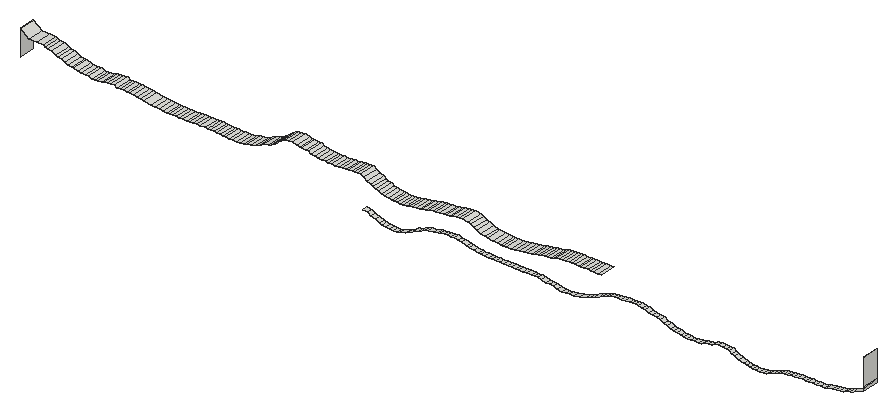
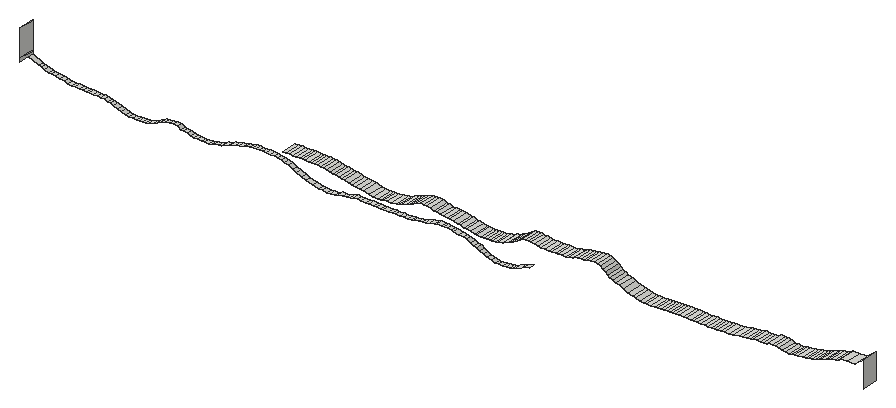
# SketchUp Ruby script. Lengths in inches.
U = 1.inch
M = Sketchup.active_model
def pt(a) = Geom::Point3d.new(a.map { |v| v * U })
def face(e, loops, mat)
  f = e.add_face(loops[0].map { |a| pt(a) })
  loops[1..].each { |l| e.add_face(l.map { |a| pt(a) }).erase! }
  f.material = f.back_material = mat if mat
  f
end
# faces: each face lists its corners as indices into pts; further lists are holes
def faces(e, pts, list, mat = nil) = list.each { |f| face(e, (f[0].is_a?(Array) ? f : [f]).map { |l| l.map { |i| pts[i] } }, mat) }
# xy, xz, yz: faces in a plane at the given z, y or x. An outline is a flat list of corners, or four numbers for a rectangle; further outlines are holes
def ring(l) = l.size == 4 ? [[l[0], l[1]], [l[2], l[1]], [l[2], l[3]], [l[0], l[3]]] : l.each_slice(2).to_a
def flat(e, list, mat, &to3) = list.each { |f| face(e, (f[0].is_a?(Array) ? f : [f]).map { |l| ring(l).map { |u, v| to3.(u, v) } }, mat) }
def xy(e, z, list, mat = nil) = flat(e, list, mat) { |x, y| [x, y, z] }
def xz(e, y, list, mat = nil) = flat(e, list, mat) { |x, z| [x, y, z] }
def yz(e, x, list, mat = nil) = flat(e, list, mat) { |y, z| [x, y, z] }
def lines(e, pts, list) = list.each { |a, b| e.add_line(pt(pts[a]), pt(pts[b])) }
# prism: a flat outline (further loops are holes) pulled along v
def prism(e, loops, v, mat = nil)
  f = face(e, loops, mat); d = Geom::Vector3d.new(v.map { |x| x * U })
  f.pushpull(f.normal.samedirection?(d) ? d.length : -d.length)
end
def box(e, o, s, mat = nil) = prism(e, [[o, [o[0] + s[0], o[1], o[2]], [o[0] + s[0], o[1] + s[1], o[2]], [o[0], o[1] + s[1], o[2]]]], [0, 0, s[2]], mat)
def at(x, y, z, deg = 0) = Geom::Transformation.translation(pt([x, y, z])) * Geom::Transformation.rotation(ORIGIN, Z_AXIS, deg.degrees)
def axes(o, x, y, z) = Geom::Transformation.new([*x, 0, *y, 0, *z, 0, *pt(o).to_a, 1])
def part(name) = M.definitions.add(name)
# library, detail: a bought-in or finely detailed component or shape, given as its bounding box
def library(name, o, s) = part(name).tap { |d| box(d.entities, o, s) }
def detail(e, o, s) = box(e.add_group.entities, o, s)
def put(e, d, t, mat = nil) = e.add_instance(d, t).tap { |i| i.material = mat if mat }
def group(e, t, mat = nil) = e.add_group.tap { |g| g.transformation = t; g.material = mat if mat }.entities
root = M.entities
xy(root,238.18,[[1254.78,565.74,1255.46,566.68]])
xy(root,238.62,[[1221.31,565.74,1222.08,566.68],[1222.08,565.74,1222.71,566.68],[1222.71,565.74,1223.47,566.68],[1223.47,565.74,1224.09,566.68],[1224.09,565.74,1224.94,566.68],
  [1224.94,565.74,1225.58,566.68],[1225.58,565.74,1226.2,566.68]])
xy(root,238.625,[[1219.89,565.74,1220.75,566.68]])
xy(root,238.89,[[1275.7,565.74,1276.38,566.68]])
xy(root,238.9,[[1277.14,565.74,1277.76,566.68],[1277.76,565.74,1278.53,566.68]])
xy(root,240.43,[[1243.98,565.74,1244.55,566.68]])
xy(root,241.68,[[1162.03,565.74,1162.62,568.68]])
xy(root,241.75,[[1164.38,565.74,1165.25,568.68],[1165.25,565.74,1165.87,568.68],[1165.87,565.74,1166.38,568.68]])
xy(root,243.05,[[1237.04,565.74,1237.72,568.68]])
xy(root,243.07,[[1235.1875,565.74,1235.77,568.68]])
xy(root,243.09,[[1231.875,565.74,1232.4,568.68],[1232.4,565.74,1232.92,568.68],[1232.92,565.74,1233.58,568.68],[1233.58,565.74,1234.03,568.68]])
yz(root,1131.59,[[565.74,241.52,568.68,246.2]])
yz(root,1285.6,[[565.74,240.89,565.74,241.29,568.68,241.52,568.68,240.89],[565.74,241.29,568.68,241.52,565.74,241.52],[565.74,241.52,565.74,246.27,566.4375,246.36,568.68,246.43,568.68,241.52],[565.74,246.27,565.74,246.43,568.68,246.43,566.4375,246.36]])
p = [[1198.39,565.74,237.11],[1198.39,566.68,237.11],[1199.15,566.68,237.04],[1199.15,565.74,237.04],[1199.84,566.68,237.01],[1199.84,565.74,237.01],
  [1200.45,566.68,236.98],[1200.45,565.74,236.98],[1201.13,566.68,237.22],[1201.13,565.74,237.22],[1197.7,565.74,237.2],[1197.7,566.68,237.2],
  [1197.17,565.74,237.33],[1197.17,566.68,237.33],[1201.98,566.68,237.43],[1201.98,565.74,237.43],[1196.5,565.74,237.68],[1196.5,566.68,237.68],
  [1202.6,566.68,237.74],[1202.6,565.74,237.74],[1265.43,565.74,237.45],[1265.43,566.68,237.45],[1266,566.68,237.42],[1266,565.74,237.42],
  [1266.73,566.68,237.4],[1266.73,565.74,237.4],[1267.41,566.68,237.47],[1267.41,565.74,237.47],[1264.24,565.74,237.59],[1264.24,566.68,237.59],
  [1264.84,566.68,237.51],[1264.84,565.74,237.51],[1268.01,566.68,237.5625],[1268.01,565.74,237.5625],[1263.7,565.74,237.71],[1263.7,566.68,237.71],
  [1268.7,566.68,237.84],[1268.7,565.74,237.84],[1195.5625,565.74,237.96],[1195.5625,566.68,237.96],[1203.3,566.68,238.02],[1203.3,565.74,238.02],
  [1230.44,565.74,237.79],[1230.44,566.68,237.79],[1231.15,566.68,237.74],[1231.15,565.74,237.74],[1232.02,566.68,237.87],[1232.02,565.74,237.87],
  [1262.87,565.74,238],[1262.87,566.68,238],[1229.67,565.74,237.86],[1229.67,566.68,237.86],[1269.38,566.68,238.08],[1269.38,565.74,238.08],
  [1229.04,565.74,238.15],[1229.04,566.68,238.15],[1232.67,566.68,237.88],[1232.67,565.74,237.88],[1233.79,566.68,238.14],[1233.79,565.74,238.14],
  [1195,565.74,238.28],[1195,566.68,238.28],[1203.74,566.68,238.375],[1203.74,565.74,238.375],[1262.16,565.74,238.33],[1262.16,566.68,238.33],
  [1228.27,565.74,238.19],[1228.27,566.68,238.19],[1235.01,566.68,238.46],[1235.01,565.74,238.46],[1252.76,565.74,238.19],[1252.76,566.68,238.19],
  [1253.58,566.68,238.15],[1253.58,565.74,238.15],[1254.11,566.68,238.11],[1254.11,565.74,238.11],[1254.78,566.68,238.18],[1254.78,565.74,238.18],
  [1270.07,566.68,238.33],[1270.07,565.74,238.33],[1227.65,565.74,238.25],[1227.65,566.68,238.25],[1252.1875,565.74,238.26],[1252.1875,566.68,238.26],
  [1255.46,565.74,238.18],[1255.46,566.68,238.18],[1256.14,566.68,238.27],[1256.14,565.74,238.27],[1194.22,565.74,238.43],[1194.22,566.68,238.43],
  [1226.89,565.74,238.45],[1226.89,566.68,238.45],[1251.62,565.74,238.48],[1251.62,566.68,238.48],[1256.66,566.68,238.55],[1256.66,565.74,238.55],
  [1261.61,565.74,238.57],[1261.61,566.68,238.57],[1270.6,566.68,238.51],[1270.6,565.74,238.51],[1204.3,566.68,238.51],[1204.3,565.74,238.51],
  [1204.9375,566.68,238.76],[1204.9375,565.74,238.76],[1226.2,565.74,238.62],[1226.2,566.68,238.62],[1235.76,566.68,238.72],[1235.76,565.74,238.72],
  [1250.96,565.74,238.56],[1250.96,566.68,238.56],[1257.32,566.68,238.61],[1257.32,565.74,238.61],[1271.17,566.68,238.6],[1271.17,565.74,238.6],
  [1217.13,565.74,238.66],[1217.13,566.68,238.66],[1217.8,566.68,238.65],[1217.8,565.74,238.65],[1218.58,566.68,238.64],[1218.58,565.74,238.64],
  [1219.2,566.68,238.63],[1219.2,565.74,238.63],[1219.89,566.68,238.625],[1219.89,565.74,238.625],[1220.75,565.74,238.625],[1220.75,566.68,238.625],
  [1221.31,566.68,238.62],[1221.31,565.74,238.62],[1250.39,565.74,238.67],[1250.39,566.68,238.67],[1257.91,566.68,238.66],[1257.91,565.74,238.66],
  [1261.11,565.74,238.86],[1261.11,566.68,238.86],[1271.83,566.68,238.74],[1271.83,565.74,238.74],[1215.29,565.74,238.78],[1215.29,566.68,238.78],
  [1215.77,566.68,238.73],[1215.77,565.74,238.73],[1216.44,566.68,238.6875],[1216.44,565.74,238.6875],[1236.64,566.68,239.08],[1236.64,565.74,239.08],
  [1249.87,565.74,239.01],[1249.87,566.68,239.01],[1258.48,566.68,239.04],[1258.48,565.74,239.04],[1272.41,566.68,238.8],[1272.41,565.74,238.8],
  [1205.58,566.68,239.12],[1205.58,565.74,239.12],[1214.41,565.74,238.93],[1214.41,566.68,238.93],[1272.98,566.68,238.83],[1272.98,565.74,238.83],
  [1273.72,566.68,238.86],[1273.72,565.74,238.86],[1213.64,565.74,239.07],[1213.64,566.68,239.07],[1260.59,565.74,238.96],[1260.59,566.68,238.96],
  [1274.48,566.68,238.875],[1274.48,565.74,238.875],[1275.02,566.68,238.88],[1275.02,565.74,238.88],[1275.7,566.68,238.89],[1275.7,565.74,238.89],
  [1276.38,565.74,238.89],[1276.38,566.68,238.89],[1277.14,566.68,238.9],[1277.14,565.74,238.9],[1278.53,565.74,238.9],[1278.53,566.68,238.9],
  [1279.16,566.68,239.15],[1279.16,565.74,239.15],[1249.1875,565.74,239.18],[1249.1875,566.68,239.18],[1259.22,566.68,239.125],[1259.22,565.74,239.125],
  [1259.9,566.68,239.02],[1259.9,565.74,239.02],[1206.16,566.68,239.22],[1206.16,565.74,239.22],[1213.09,565.74,239.16],[1213.09,566.68,239.16],
  [1237.43,566.68,239.375],[1237.43,565.74,239.375],[1207.16,566.68,239.31],[1207.16,565.74,239.31],[1212.24,565.74,239.44],[1212.24,566.68,239.44],
  [1248.5625,565.74,239.5],[1248.5625,566.68,239.5],[1279.93,566.68,239.28],[1279.93,565.74,239.28],[1207.97,566.68,239.54],[1207.97,565.74,239.54],
  [1280.73,566.68,239.42],[1280.73,565.74,239.42],[1211.57,565.74,239.56],[1211.57,566.68,239.56],[1238.17,566.68,239.75],[1238.17,565.74,239.75],
  [1281.45,566.68,239.49],[1281.45,565.74,239.49],[1208.46,566.68,239.6],[1208.46,565.74,239.6],[1247.8,565.74,239.65],[1247.8,566.68,239.65],
  [1282,566.68,239.53],[1282,565.74,239.53],[1282.6875,566.68,239.81],[1282.6875,565.74,239.81],[1209.08,566.68,239.65],[1209.08,565.74,239.65],
  [1209.67,566.68,239.69],[1209.67,565.74,239.69],[1210.96,565.74,239.72],[1210.96,566.68,239.72],[1210.23,566.68,239.7],[1210.23,565.74,239.7],
  [1238.82,566.68,239.97],[1238.82,565.74,239.97],[1247.1875,565.74,239.8],[1247.1875,566.68,239.8],[1246.43,565.74,239.96],[1246.43,566.68,239.96],
  [1283.21,566.68,239.96],[1283.21,565.74,239.96],[1239.44,566.68,240.17],[1239.44,565.74,240.17],[1245.78,565.74,240.23],[1245.78,566.68,240.23],
  [1283.77,566.68,240.1],[1283.77,565.74,240.1],[1285.6,566.68,240.89],[1285.6,565.74,240.89],[1240.12,566.68,240.27],[1240.12,565.74,240.27],
  [1245.2,565.74,240.27],[1245.2,566.68,240.27],[1240.8,566.68,240.33],[1240.8,565.74,240.33],[1241.49,566.68,240.37],[1241.49,565.74,240.37],
  [1244.55,565.74,240.43],[1244.55,566.68,240.43],[1242.18,566.68,240.4],[1242.18,565.74,240.4],[1242.875,566.68,240.41],[1242.875,565.74,240.41],
  [1243.4,566.68,240.42],[1243.4,565.74,240.42],[1243.98,566.68,240.43],[1243.98,565.74,240.43],[1168.01,568.68,241.57],[1168.55,568.68,241.53],
  [1168.55,565.74,241.53],[1168.01,565.74,241.57],[1169.17,568.68,241.51],[1169.17,565.74,241.51],[1169.72,568.68,241.49],[1169.72,565.74,241.49],
  [1170.42,568.68,241.48],[1170.42,565.74,241.48],[1171.08,568.68,241.47],[1171.08,565.74,241.47],[1171.65,568.68,241.46],[1171.65,565.74,241.46],
  [1172.36,568.68,241.6],[1172.36,565.74,241.6],[1218.73,568.68,241.56],[1219.33,568.68,241.51],[1219.33,565.74,241.51],[1218.73,565.74,241.56],
  [1219.78,568.68,241.48],[1219.78,565.74,241.48],[1220.3,568.68,241.46],[1220.3,565.74,241.46],[1221.17,568.68,241.51],[1221.17,565.74,241.51],
  [1221.89,568.68,241.59],[1221.89,565.74,241.59],[1167.4,568.68,241.66],[1167.4,565.74,241.66],[1173.09,568.68,241.85],[1173.09,565.74,241.85],
  [1216.91,568.68,241.78],[1217.96,568.68,241.63],[1217.96,565.74,241.63],[1216.91,565.74,241.78],[1222.83,568.68,241.82],[1222.83,565.74,241.82],
  [1158.37,568.68,241.75],[1158.82,568.68,241.74],[1158.82,565.74,241.74],[1158.37,565.74,241.75],[1159.37,568.68,241.72],[1159.37,565.74,241.72],
  [1160,568.68,241.71],[1160,565.74,241.71],[1160.63,568.68,241.7],[1160.63,565.74,241.7],[1161.36,568.68,241.69],[1161.36,565.74,241.69],
  [1162.03,568.68,241.68],[1162.03,565.74,241.68],[1162.62,568.68,241.68],[1163.11,568.68,241.67],[1163.11,565.74,241.67],[1162.62,565.74,241.68],
  [1163.8125,568.68,241.74],[1163.8125,565.74,241.74],[1164.38,568.68,241.75],[1164.38,565.74,241.75],[1166.38,568.68,241.75],[1166.87,568.68,241.67],
  [1166.87,565.74,241.67],[1166.38,565.74,241.75],[1156.18,568.68,241.89],[1157,568.68,241.83],[1157,565.74,241.83],[1156.18,565.74,241.89],
  [1157.6,568.68,241.78],[1157.6,565.74,241.78],[1173.76,568.68,241.91],[1173.76,565.74,241.91],[1199.39,568.68,241.89],[1199.85,568.68,241.85],
  [1199.85,565.74,241.85],[1199.39,565.74,241.89],[1200.37,568.68,241.8125],[1200.37,565.74,241.8125],[1200.88,568.68,241.79],[1200.88,565.74,241.79],
  [1201.46,568.68,241.78],[1201.46,565.74,241.78],[1202.13,568.68,241.91],[1202.13,565.74,241.91],[1216.42,568.68,241.89],[1216.42,565.74,241.89],
  [1223.61,568.68,241.87],[1223.61,565.74,241.87],[1155.41,568.68,241.96],[1155.41,565.74,241.96],[1174.66,568.68,242.1],[1174.66,565.74,242.1],
  [1198.83,568.68,241.96],[1198.83,565.74,241.96],[1202.6,568.68,241.93],[1202.6,565.74,241.93],[1203.27,568.68,242.09],[1203.27,565.74,242.09],
  [1215.78,568.68,242.14],[1215.78,565.74,242.14],[1224.375,568.68,241.98],[1224.375,565.74,241.98],[1154.24,568.68,242.24],[1154.24,565.74,242.24],
  [1198.15,568.68,242.11],[1198.15,565.74,242.11],[1224.99,568.68,242.02],[1224.99,565.74,242.02],[1225.64,568.68,242.19],[1225.64,565.74,242.19],
  [1175.43,568.68,242.46],[1175.43,565.74,242.46],[1197.55,568.68,242.21],[1197.55,565.74,242.21],[1204.04,568.68,242.2],[1204.04,565.74,242.2],
  [1215.02,568.68,242.39],[1215.02,565.74,242.39],[1153.57,568.68,242.34],[1153.57,565.74,242.34],[1197.04,568.68,242.51],[1197.04,565.74,242.51],
  [1204.54,568.68,242.24],[1204.54,565.74,242.24],[1205.15,568.68,242.42],[1205.15,565.74,242.42],[1226.34,568.68,242.38],[1226.34,565.74,242.38],
  [1152.91,568.68,242.38],[1152.91,565.74,242.38],[1152.25,568.68,242.48],[1152.25,565.74,242.48],[1205.7,568.68,242.47],[1205.7,565.74,242.47],
  [1214.4,568.68,242.65],[1214.4,565.74,242.65],[1226.83,568.68,242.4375],[1226.83,565.74,242.4375],[1227.35,568.68,242.48],[1227.35,565.74,242.48],
  [1144.07,568.68,242.68],[1144.74,568.68,242.51],[1144.74,565.74,242.51],[1144.07,565.74,242.68],[1145.26,568.68,242.46],[1145.26,565.74,242.46],
  [1145.8,568.68,242.58],[1145.8,565.74,242.58],[1151.61,568.68,242.57],[1151.61,565.74,242.57],[1176.13,568.68,242.78],[1176.13,565.74,242.78],
  [1196.45,568.68,242.68],[1196.45,565.74,242.68],[1206.45,568.68,242.71],[1206.45,565.74,242.71],[1228.01,568.68,242.58],[1228.01,565.74,242.58],
  [1146.43,568.68,242.57],[1146.43,565.74,242.57],[1147.06,568.68,242.81],[1147.06,565.74,242.81],[1148.83,568.68,242.92],[1149.26,568.68,242.625],
  [1149.26,565.74,242.625],[1148.83,565.74,242.92],[1149.87,568.68,242.65],[1149.87,565.74,242.65],[1150.42,568.68,242.62],[1150.42,565.74,242.62],
  [1151.05,568.68,242.58],[1151.05,565.74,242.58],[1213.85,568.68,242.9375],[1213.85,565.74,242.9375],[1228.54,568.68,242.61],[1228.54,565.74,242.61],
  [1229.125,568.68,242.77],[1229.125,565.74,242.77],[1142.72,568.68,242.78],[1143.53,568.68,242.73],[1143.53,565.74,242.73],[1142.72,565.74,242.78],
  [1195.95,568.68,242.875],[1195.95,565.74,242.875],[1207.09,568.68,242.78],[1207.09,565.74,242.78],[1141.42,568.68,243.06],[1142.14,568.68,242.85],
  [1142.14,565.74,242.85],[1141.42,565.74,243.06],[1147.63,568.68,242.86],[1147.63,565.74,242.86],[1176.9,568.68,242.97],[1176.9,565.74,242.97],
  [1207.57,568.68,242.82],[1207.57,565.74,242.82],[1208.26,568.68,242.85],[1208.26,565.74,242.85],[1229.58,568.68,242.95],[1229.58,565.74,242.95],
  [1148.19,568.68,242.89],[1148.19,565.74,242.89],[1195.56,568.68,243.09],[1195.56,565.74,243.09],[1208.96,568.68,242.87],[1208.96,565.74,242.87],
  [1209.51,568.68,243.02],[1209.51,565.74,243.02],[1213.28,568.68,243.14],[1213.28,565.74,243.14],[1177.43,568.68,243.23],[1177.43,565.74,243.23],
  [1210.13,568.68,243.05],[1210.13,565.74,243.05],[1230.14,568.68,243.01],[1230.14,565.74,243.01],[1230.65,568.68,243.05],[1230.65,565.74,243.05],
  [1231.22,568.68,243.08],[1231.22,565.74,243.08],[1140.35,568.68,243.3],[1140.9375,568.68,243.14],[1140.9375,565.74,243.14],[1140.35,565.74,243.3],
  [1194.95,568.68,243.43],[1194.95,565.74,243.43],[1210.68,568.68,243.29],[1210.68,565.74,243.29],[1212.51,568.68,243.42],[1212.51,565.74,243.42],
  [1231.875,568.68,243.09],[1231.875,565.74,243.09],[1234.03,568.68,243.09],[1234.6,568.68,243.08],[1234.6,565.74,243.08],[1234.03,565.74,243.09],
  [1235.1875,568.68,243.07],[1235.1875,565.74,243.07],[1235.77,568.68,243.07],[1236.43,568.68,243.0625],[1236.43,565.74,243.0625],[1235.77,565.74,243.07],
  [1237.04,568.68,243.05],[1237.04,565.74,243.05],[1177.83,568.68,243.48],[1177.83,565.74,243.48],[1139.71,568.68,243.48],[1139.71,565.74,243.48],
  [1211.36,568.68,243.35],[1211.36,565.74,243.35],[1194.41,568.68,243.8],[1194.41,565.74,243.8],[1211.91,568.68,243.39],[1211.91,565.74,243.39],
  [1139.19,568.68,243.79],[1139.19,565.74,243.79],[1178.35,568.68,243.72],[1178.35,565.74,243.72],[1178.6875,568.68,244.12],[1178.6875,565.74,244.12],
  [1138.53,568.68,243.95],[1138.53,565.74,243.95],[1193.81,568.68,244.18],[1193.81,565.74,244.18],[1138.01,568.68,244.11],[1138.01,565.74,244.11],
  [1186.63,568.68,243.99],[1187.35,568.68,243.95],[1187.35,565.74,243.95],[1186.63,565.74,243.99],[1187.85,568.68,243.93],[1187.85,565.74,243.93],
  [1188.54,568.68,243.91],[1188.54,565.74,243.91],[1189.11,568.68,243.89],[1189.11,565.74,243.89],[1189.81,568.68,243.88],[1189.81,565.74,243.88],
  [1190.46,568.68,243.94],[1190.46,565.74,243.94],[1191.1,568.68,243.95],[1191.1,565.74,243.95],[1191.66,568.68,244.1],[1191.66,565.74,244.1],
  [1185.45,568.68,244.11],[1186.01,568.68,244.04],[1186.01,565.74,244.04],[1185.45,565.74,244.11],[1137.34,568.68,244.41],[1137.34,565.74,244.41],
  [1179.16,568.68,244.39],[1179.16,565.74,244.39],[1184.7,568.68,244.25],[1184.7,565.74,244.25],[1192.29,568.68,244.13],[1192.29,565.74,244.13],
  [1192.77,568.68,244.15],[1192.77,565.74,244.15],[1193.29,568.68,244.17],[1193.29,565.74,244.17],[1184.24,568.68,244.51],[1184.24,565.74,244.51],
  [1136.58,568.68,244.54],[1136.58,565.74,244.54],[1179.64,568.68,244.73],[1179.64,565.74,244.73],[1136.02,568.68,244.61],[1136.02,565.74,244.61],
  [1183.09,568.68,244.67],[1183.7,568.68,244.55],[1183.7,565.74,244.55],[1183.09,565.74,244.67],[1135.8,568.68,244.92],[1135.8,565.74,244.92],
  [1180.125,568.68,244.87],[1180.125,565.74,244.87],[1182.04,568.68,244.81],[1182.61,568.68,244.7],[1182.61,565.74,244.7],[1182.04,565.74,244.81],
  [1181.39,568.68,245.01],[1181.39,565.74,245.01],[1133.16,568.68,244.96],[1134.55,568.68,244.9375],[1134.55,565.74,244.9375],[1133.16,565.74,244.96],
  [1180.71,568.68,244.95],[1180.71,565.74,244.95],[1131.59,568.68,246.2],[1131.59,565.74,246.2]]
faces(root,p,[[0,1,2,3],[3,2,4,5],[5,4,6,7],[7,6,8,9],[10,11,1,0],[12,13,11,10],[9,8,14,15],[16,17,13,12],
  [15,14,18,19],[20,21,22,23],[23,22,24,25],[25,24,26,27],[28,29,30,31],[31,30,21,20],[27,26,32,33],[34,35,29,28],
  [33,32,36,37],[38,39,17,16],[19,18,40,41],[42,43,44,45],[45,44,46,47],[48,49,35,34],[50,51,43,42],[37,36,52,53],
  [54,55,51,50],[47,46,56,57],[57,56,58,59],[60,61,39,38],[41,40,62,63],[64,65,49,48],[66,67,55,54],[59,58,68,69],
  [70,71,72,73],[73,72,74,75],[75,74,76,77],[53,52,78,79],[80,81,67,66],[82,83,71,70],[84,85,86,87],[88,89,61,60],
  [90,91,81,80],[92,93,83,82],[87,86,94,95],[96,97,65,64],[79,78,98,99],[63,62,100,101],[101,100,102,103],[104,105,91,90],
  [69,68,106,107],[108,109,93,92],[95,94,110,111],[99,98,112,113],[114,115,116,117],[117,116,118,119],[119,118,120,121],[121,120,122,123],
  [124,125,126,127],[128,129,109,108],[111,110,130,131],[132,133,97,96],[113,112,134,135],[136,137,138,139],[139,138,140,141],[141,140,115,114],
  [107,106,142,143],[144,145,129,128],[131,130,146,147],[135,134,148,149],[103,102,150,151],[152,153,137,136],[149,148,154,155],[155,154,156,157],
  [158,159,153,152],[160,161,133,132],[157,156,162,163],[163,162,164,165],[165,164,166,167],[168,169,170,171],[172,173,174,175],[176,177,145,144],
  [147,146,178,179],[179,178,180,181],[181,180,161,160],[151,150,182,183],[184,185,159,158],[143,142,186,187],[183,182,188,189],[190,191,185,184],
  [192,193,177,176],[175,174,194,195],[189,188,196,197],[195,194,198,199],[200,201,191,190],[187,186,202,203],[199,198,204,205],[197,196,206,207],
  [208,209,193,192],[205,204,210,211],[211,210,212,213],[207,206,214,215],[215,214,216,217],[218,219,201,200],[217,216,220,221],[221,220,219,218],
  [203,202,222,223],[224,225,209,208],[226,227,225,224],[213,212,228,229],[223,222,230,231],[232,233,227,226],[229,228,234,235],[235,234,236,237],
  [231,230,238,239],[240,241,233,232],[239,238,242,243],[243,242,244,245],[246,247,241,240],[245,244,248,249],[249,248,250,251],[251,250,252,253],
  [253,252,254,255],[256,257,258,259],[257,260,261,258],[260,262,263,261],[262,264,265,263],[264,266,267,265],[266,268,269,267],[268,270,271,269],
  [272,273,274,275],[273,276,277,274],[276,278,279,277],[278,280,281,279],[280,282,283,281],[284,256,259,285],[270,286,287,271],[288,289,290,291],
  [289,272,275,290],[282,292,293,283],[294,295,296,297],[295,298,299,296],[298,300,301,299],[300,302,303,301],[302,304,305,303],[304,306,307,305],
  [308,309,310,311],[309,312,313,310],[312,314,315,313],[316,317,318,319],[317,284,285,318],[320,321,322,323],[321,324,325,322],[324,294,297,325],
  [286,326,327,287],[328,329,330,331],[329,332,333,330],[332,334,335,333],[334,336,337,335],[336,338,339,337],[340,288,291,341],[292,342,343,293],
  [344,320,323,345],[326,346,347,327],[348,328,331,349],[338,350,351,339],[350,352,353,351],[354,340,341,355],[342,356,357,343],[358,344,345,359],
  [360,348,349,361],[356,362,363,357],[362,364,365,363],[346,366,367,347],[368,360,361,369],[352,370,371,353],[372,354,355,373],[374,358,359,375],
  [376,368,369,377],[370,378,379,371],[378,380,381,379],[364,382,383,365],[384,374,375,385],[386,384,385,387],[380,388,389,381],[390,372,373,391],
  [382,392,393,383],[392,394,395,393],[396,397,398,399],[397,400,401,398],[400,402,403,401],[404,386,387,405],[366,406,407,367],[408,376,377,409],
  [388,410,411,389],[394,412,413,395],[402,414,415,403],[414,416,417,415],[418,419,420,421],[419,422,423,420],[422,424,425,423],[424,426,427,425],
  [426,404,405,427],[428,390,391,429],[412,430,431,413],[430,432,433,431],[434,435,436,437],[435,396,399,436],[438,408,409,439],[410,440,441,411],
  [442,443,444,445],[443,434,437,444],[416,446,447,417],[406,448,449,407],[440,450,451,441],[450,452,453,451],[432,454,455,433],[446,456,457,447],
  [456,418,421,457],[458,438,439,459],[452,460,461,453],[460,462,463,461],[464,428,429,465],[448,466,467,449],[462,468,469,463],[454,470,471,455],
  [470,472,473,471],[472,474,475,473],[476,477,478,479],[477,442,445,478],[480,458,459,481],[468,482,483,469],[484,464,465,485],[474,486,487,475],
  [488,489,490,491],[489,492,493,490],[494,495,496,497],[495,498,499,496],[466,500,501,467],[502,476,479,503],[482,504,505,483],[506,480,481,507],
  [504,508,509,505],[508,484,485,509],[510,502,503,511],[500,512,513,501],[512,514,515,513],[516,510,511,517],[518,506,507,519],[520,516,517,521],
  [522,523,524,525],[523,526,527,524],[526,528,529,527],[528,530,531,529],[530,532,533,531],[532,534,535,533],[534,536,537,535],[536,538,539,537],
  [540,541,542,543],[541,522,525,542],[544,520,521,545],[514,546,547,515],[548,540,543,549],[538,550,551,539],[550,552,553,551],[552,554,555,553],
  [554,518,519,555],[556,548,549,557],[558,544,545,559],[546,560,561,547],[562,558,559,563],[564,565,566,567],[565,556,557,566],[568,562,563,569],
  [560,570,571,561],[572,573,574,575],[573,564,567,574],[576,572,575,577],[578,579,580,581],[579,568,569,580],[570,582,583,571],[582,576,577,583],
  [584,578,581,585]])
